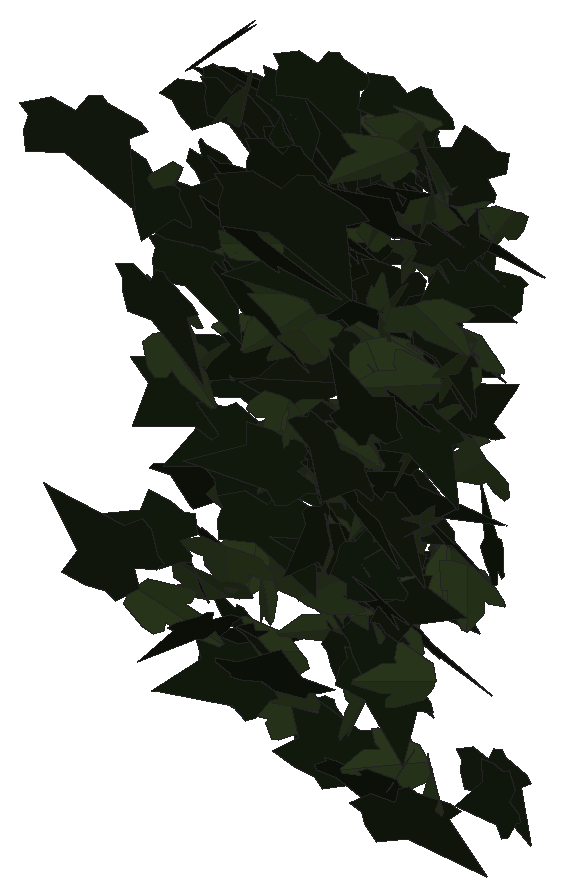
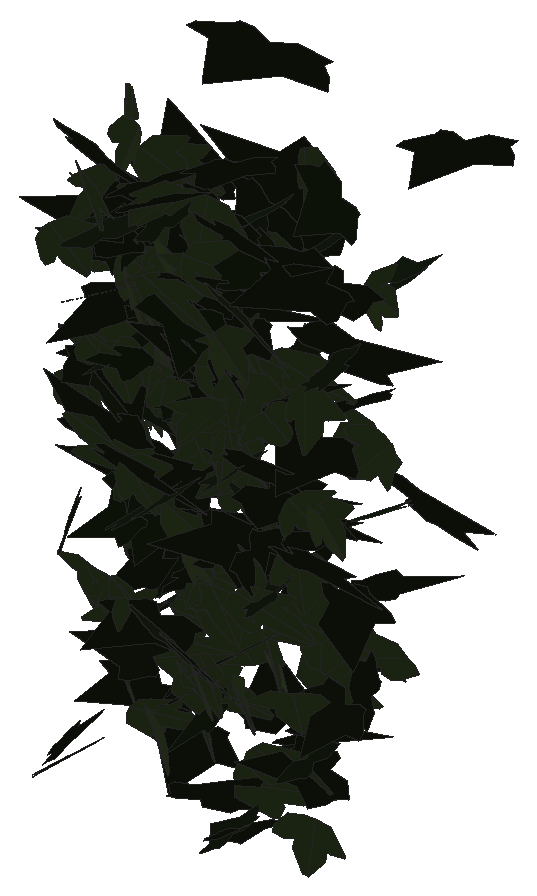
# SketchUp Ruby script. Lengths in millimetres.
U = 1.mm
M = Sketchup.active_model
def pt(a) = Geom::Point3d.new(a.map { |v| v * U })
def face(e, loops, mat)
  f = e.add_face(loops[0].map { |a| pt(a) })
  loops[1..].each { |l| e.add_face(l.map { |a| pt(a) }).erase! }
  f.material = f.back_material = mat if mat
  f
end
# faces: each face lists its corners as indices into pts; further lists are holes
def faces(e, pts, list, mat = nil) = list.each { |f| face(e, (f[0].is_a?(Array) ? f : [f]).map { |l| l.map { |i| pts[i] } }, mat) }
# xy, xz, yz: faces in a plane at the given z, y or x. An outline is a flat list of corners, or four numbers for a rectangle; further outlines are holes
def ring(l) = l.size == 4 ? [[l[0], l[1]], [l[2], l[1]], [l[2], l[3]], [l[0], l[3]]] : l.each_slice(2).to_a
def flat(e, list, mat, &to3) = list.each { |f| face(e, (f[0].is_a?(Array) ? f : [f]).map { |l| ring(l).map { |u, v| to3.(u, v) } }, mat) }
def xy(e, z, list, mat = nil) = flat(e, list, mat) { |x, y| [x, y, z] }
def xz(e, y, list, mat = nil) = flat(e, list, mat) { |x, z| [x, y, z] }
def yz(e, x, list, mat = nil) = flat(e, list, mat) { |y, z| [x, y, z] }
def lines(e, pts, list) = list.each { |a, b| e.add_line(pt(pts[a]), pt(pts[b])) }
# prism: a flat outline (further loops are holes) pulled along v
def prism(e, loops, v, mat = nil)
  f = face(e, loops, mat); d = Geom::Vector3d.new(v.map { |x| x * U })
  f.pushpull(f.normal.samedirection?(d) ? d.length : -d.length)
end
def box(e, o, s, mat = nil) = prism(e, [[o, [o[0] + s[0], o[1], o[2]], [o[0] + s[0], o[1] + s[1], o[2]], [o[0], o[1] + s[1], o[2]]]], [0, 0, s[2]], mat)
def at(x, y, z, deg = 0) = Geom::Transformation.translation(pt([x, y, z])) * Geom::Transformation.rotation(ORIGIN, Z_AXIS, deg.degrees)
def axes(o, x, y, z) = Geom::Transformation.new([*x, 0, *y, 0, *z, 0, *pt(o).to_a, 1])
def part(name) = M.definitions.add(name)
# library, detail: a bought-in or finely detailed component or shape, given as its bounding box
def library(name, o, s) = part(name).tap { |d| box(d.entities, o, s) }
def detail(e, o, s) = box(e.add_group.entities, o, s)
def put(e, d, t, mat = nil) = e.add_instance(d, t).tap { |i| i.material = mat if mat }
def group(e, t, mat = nil) = e.add_group.tap { |g| g.transformation = t; g.material = mat if mat }.entities
root = M.entities
M.materials.add("efeu1").color = [18, 25, 13]
M.materials.add("efeu2").color = [43, 57, 29]
c1 = part("ivyleaf_10")
p = [[0,12.8,-0.8],[-1.5,51.3,-10.9],[-4.9,51,-11.6],[-13.6,26.5,-7.3],[-13.2,15.9,-4.6],[-21.1,19.3,-7.2],
  [-29.5,16.3,-8.3],[-29.2,8.3,-6.2],[-19.7,-9.8,0.5],[-7.6,-13,4],[1,-12.2,5.8],[-0.4,51.1,-11.1],
  [-1.5,51.1,-10.9],[1,-12.4,5.9],[16.9,-12.4,3.5],[35.1,9.1,-5.1],[35,12.9,-6.1],[20.5,16.4,-4.9],
  [15.8,15,-3.8],[15.3,27.6,-7.1],[12.8,31.3,-7.8]]
faces(c1.entities,p,[[0,1,2,3,4,5,6,7,8,9,10],[11,12,0,13,14,15,16,17,18,19,20]],"efeu2")
c2 = part("ivyleaf_9")
p = [[39.1,54.8,31.7],[34.5,51.8,30.2],[-5.3,25.2,17.3],[-17.9,28.3,20.9],[-21.6,21.7,17],[-20.2,4.3,5.3],
  [-22.9,-0.3,2.5],[-17.1,-4,-0.6],[-2,-2.1,-1.2],[-0.7,-15.4,-10.1],[16.6,-22.3,-16.7],[21.1,-15.1,-12.5],
  [32.7,-10.7,-11],[46.1,-1.8,-6.6],[30.8,11.2,3.8]]
faces(c2.entities,p,[[0,1,2,3,4,5,6,7,8,9,10,11,12,13,14]],"efeu1")
put(root,c1,axes([4543,678,3138.6],[-1.58193,0.83154,-0.42194],[0.58084,-0.2915,-1.17569],[-1.67692,-0.88541,-0.00919]))
put(root,c2,axes([4588.4,773.9,3017.7],[-2.04189,0.02362,0.17491],[-0.33312,-0.00391,-1.0731],[-0.04317,-1.08703,0.00766]))
put(root,c2,axes([4606.5,683.4,3248.6],[-0.26226,0.22071,1.22906],[-2.23046,0.404,-0.20395],[-0.8204,-1.16891,0.16157]))
put(root,c2,axes([4552.5,734,2811.4],[1.82354,-0.20517,-0.47825],[-0.87023,0.14656,-0.97893],[0.47292,1.06079,0.04275]))
put(root,c2,axes([4543.6,748.2,3283.7],[1.23051,-0.828,-0.4397],[-0.38091,0.39991,-1.04736],[1.74312,0.67189,0.08152]))
put(root,c1,axes([4575.2,767.9,2648.4],[-1.90726,0.31844,0.17004],[-0.30872,0.051,-1.05151],[-0.61377,-1.01518,0.00051]))
put(root,c2,axes([4537.2,702.8,2816.5],[0.74967,-0.34619,-1.19939],[2.1006,-0.49105,0.50421],[-1.11007,-1.163,0.14414]))
put(root,c2,axes([4581.6,675.2,3027.2],[-1.24627,-0.64137,0.7681],[-0.4534,-0.79163,-0.86412],[1.8497,-0.62618,0.3057]))
put(root,c1,axes([4579.2,767.7,3230.3],[-0.5778,-1.08084,-0.38707],[0.14495,0.38054,-1.12231],[2.18017,-0.31175,-0.02797]))
put(root,c1,axes([4585.8,734,3058.8],[-0.07425,-1.08579,0.28514],[-0.03125,-0.28473,-1.08647],[2.13631,-0.0419,-0.00598]))
put(root,c2,axes([4552.8,739.9,3387.1],[0.13799,-0.32705,-1.15112],[0.68535,1.10574,-0.29147],[2.17196,-0.32813,0.16511]))
put(root,c1,axes([4580.9,639.1,3320.3],[0.20368,-0.86346,0.89476],[0.52681,-0.85899,-0.86205],[2.30715,0.27237,0.11785]))
put(root,c2,axes([4566.5,488.5,3464.7],[-0.43438,-1.01787,-0.89838],[0.34428,0.88006,-1.04307],[2.5608,-0.29098,-0.01215]))
put(root,c2,axes([4575.9,613.6,3327.7],[-0.59648,-0.98235,0.68898],[0.03231,-0.71566,-1.01265],[2.28337,-0.24649,0.19431]))
put(root,c2,axes([4599.1,686,2926.4],[1.22379,0.74994,-0.59671],[-0.79032,-0.42959,-0.98739],[-1.64384,0.76484,0.03049]))
put(root,c2,axes([4618.7,599.2,2886.3],[-0.86103,-0.01575,1.0083],[-1.64942,-0.55895,-0.39759],[0.98126,-0.95338,0.21644]))
put(root,c2,axes([4570.8,692.8,3200.3],[0.10671,-1.19416,-0.39132],[0.1469,0.39424,-1.19202],[2.38712,0.02912,0.09085]))
put(root,c2,axes([4586.6,736.4,3163.5],[1.65295,0.72592,0.00561],[0.0086,0.00335,-1.13194],[-1.3816,0.86852,-0.00033]))
put(root,c2,axes([4564.4,759.5,3393.3],[2.16142,0.05518,0.26359],[0.50154,0.00784,-1.13701],[-0.10567,1.16584,-0.00483]))
put(root,c2,axes([4595.4,689.4,3465.5],[0.63579,0.74247,0.95484],[0.67931,0.88596,-0.81379],[-2.19947,0.48825,0.02467]))
put(root,c1,axes([4599.4,762.2,3076.5],[-0.59048,-0.8322,0.71685],[0.42812,-0.77725,-0.80496],[2.04612,-0.07753,0.3753]))
put(root,c1,axes([4621.6,673.6,2786.3],[-1.68313,-0.18792,-0.61587],[-0.96086,-0.44705,0.86138],[-0.76061,0.98059,0.27467]))
put(root,c1,axes([4623.6,727.9,2973.4],[-1.052,-0.93491,-0.06473],[0.04904,0.05996,-1.08606],[1.7829,-0.55329,-0.00832]))
put(root,c2,axes([4613.3,748.2,3215.6],[-0.75152,-1.04404,0.26644],[-0.20737,-0.24363,-1.11612],[2.0402,-0.40934,-0.0153]))
put(root,c1,axes([4613.3,749.5,2803.8],[1.57621,0.62267,-0.15147],[-0.20029,-0.11201,-1.03583],[-1.20306,0.83445,-0.02601]))
put(root,c2,axes([4665.5,458.4,2930.9],[-2.06405,0.06241,-0.80267],[-1.52815,0.01453,1.08601],[0.11193,1.34916,0.02543]))
put(root,c2,axes([4598.8,707.9,2695.6],[0.35202,0.71468,-0.82032],[0.0774,0.82697,0.72964],[2.06919,-0.15252,0.11226]))
put(root,c1,axes([4613.4,726.1,3186.5],[-0.63082,1.06439,-0.19666],[0.13514,-0.18385,-1.11473],[-2.0556,-0.33872,-0.01293]))
put(root,c1,axes([4657.8,718.8,3229],[0.93414,0.12753,-1.01683],[-1.92982,-0.10292,-0.50236],[-0.2826,1.1244,0.06935]))
put(root,c1,axes([4598.7,741.9,3218.9],[-0.82622,0.33455,-1.04055],[1.21718,-0.83021,-0.53374],[-1.68695,-0.76287,0.12453]))
put(root,c1,axes([4588.3,626.6,3111.4],[1.34835,-0.17595,0.94708],[1.77036,-0.1805,-0.72937],[0.47634,1.16889,0.02993]))
put(root,c2,axes([4648,747.1,3075.7],[-0.01518,0.23814,-1.12079],[-0.44844,-1.0972,-0.23145],[-2.1341,0.22887,0.05661]))
put(root,c1,axes([4633.6,776.7,3192.4],[0.54211,0.89749,-0.56787],[-0.73234,-0.46079,-0.92125],[-1.88397,0.43737,0.19471]))
put(root,c2,axes([4597,739,2721.3],[0.71859,-0.97928,0.3703],[0.41503,-0.31145,-1.046],[1.94886,0.42741,0.08622]))
put(root,c1,axes([4591.2,592.3,2800.7],[0.8964,0.2162,0.97025],[1.6901,0.39094,-0.5182],[-0.85013,1.00518,-0.00715]))
put(root,c2,axes([4606.6,718.4,3400.2],[0.47706,-1.1436,0.04901],[0.00765,-0.04929,-1.17073],[2.17849,0.2506,-0.00662]))
put(root,c1,axes([4666.3,733.7,2698.9],[-0.98064,0.01279,0.89908],[-1.47187,-0.53494,-0.4356],[0.87303,-0.88751,0.27551]))
put(root,c1,axes([4645.7,661,2848.3],[-2.04059,-0.16162,0.08184],[-0.15185,-0.01977,-1.08427],[0.30954,-1.07513,0.00763]))
put(root,c2,axes([4661.4,677.6,2998.2],[-1.70018,-0.43925,0.45376],[-0.66037,-0.31541,-0.98843],[1.00428,-0.95103,0.11824]))
put(root,c1,axes([4672.6,759,2918.6],[-1.02752,-0.21117,0.91697],[-1.42909,-0.54043,-0.56656],[1.07927,-0.91665,0.12279]))
put(root,c1,axes([4620,711.2,2884.1],[-0.68337,-0.57703,0.9887],[1.15406,0.78302,0.67721],[-1.84796,0.70238,0.0573]))
put(root,c2,axes([4673.6,664.4,2697.8],[-1.32992,-0.4501,0.85865],[-1.25427,-0.55574,-0.82765],[1.35322,-0.95746,0.07674]))
put(root,c2,axes([4687.5,774.7,3119.1],[-2.04699,-0.09835,0.22206],[-0.41345,-0.06118,-1.07929],[0.20666,-1.09653,0.0403]))
put(root,c1,axes([4699.2,715.9,2644.9],[-0.06533,0.03688,-1.24408],[-2.21027,-0.44855,0.01875],[-0.85192,1.16091,0.04677]))
put(root,c2,axes([4680.6,582.9,2808.3],[-0.57562,0.60142,-0.88442],[0.19749,-0.89826,-0.64632],[-2.02593,-0.25844,0.18828]))
put(root,c2,axes([4634.2,737.6,3362.5],[0.96968,-1.08808,0.14521],[0.11602,-0.1318,-1.20146],[2.08597,0.51313,-0.00068]))
put(root,c2,axes([4649.5,680.5,2954.9],[0.60981,-0.95034,-0.85727],[-0.55424,0.80641,-1.00281],[2.37195,0.43275,-0.01392]))
put(root,c2,axes([4641.8,754.4,2944.4],[1.04178,-0.96438,-0.08653],[-0.04623,0.08569,-1.1087],[1.8422,0.54752,0.02111]))
put(root,c2,axes([4642.7,527.9,3253.3],[0.68393,-1.31283,-0.03189],[-0.01948,0.03026,-1.36113],[2.49924,0.3595,-0.00188]))
put(root,c1,axes([4672.4,767.1,3220.9],[-1.07092,-0.94805,-0.32511],[0.41799,0.24715,-1.10082],[1.86112,-0.60103,0.06016]))
put(root,c2,axes([4680.7,743.6,2979.8],[-0.47406,0.25077,-1.09909],[0.74862,-1.03553,-0.32541],[-2.01071,-0.44467,0.13797]))
put(root,c1,axes([4678.5,713.4,2845.2],[0.89008,-0.92506,-0.4502],[-0.1471,0.46154,-1.02866],[1.95246,0.45648,0.12773]))
put(root,c1,axes([4670.1,781.1,2803.5],[0.94415,-0.91619,0.26202],[0.28525,-0.2167,-1.04151],[1.79103,0.51749,0.02775]))
put(root,c1,axes([4678.1,643.1,3464.8],[0.02137,-1.16228,-0.38586],[0.1283,0.38588,-1.16037],[2.32722,-0.0106,0.06751]))
put(root,c1,axes([4661.2,713.2,2788.2],[-0.56556,0.049,-1.06746],[0.45682,-1.07659,-0.11624],[-1.98176,-0.26215,0.27784]))
put(root,c1,axes([4700.3,697.4,3195.4],[-1.21986,-0.81554,0.40318],[-0.50925,-0.30239,-1.03704],[1.65487,-0.69421,-0.02193]))
put(root,c2,axes([4674.6,772.7,2617.8],[-0.51151,-0.98309,0.00849],[0.00873,-0.01006,-1.01914],[1.87107,-0.26871,0.00708]))
put(root,c1,axes([4695.2,783.7,3272.6],[-0.06078,-1.05145,0.41917],[0.0409,-0.41982,-1.05145],[2.15388,-0.0217,0.03179]))
put(root,c2,axes([4724.8,752.1,3317.8],[-1.07947,0.89986,0.44017],[-0.51038,0.35098,-1.06306],[-1.83694,-0.62631,0.0367]))
put(root,c2,axes([4660.8,650.3,3213.9],[1.55261,-1.023,-0.08756],[-0.09223,0.07335,-1.30842],[1.95191,0.81719,0.00782]))
put(root,c1,axes([4698.4,727.9,2958],[0.01329,-0.3992,1.07691],[0.09042,-1.07591,-0.39914],[2.18399,0.04697,0.00997]))
put(root,c1,axes([4691.6,703.7,3187.5],[0.23506,-0.31709,-1.15718],[0.66422,1.12249,-0.27033],[2.1848,-0.30714,0.20669]))
put(root,c2,axes([4722,757.2,3411.1],[-2.19236,0.12858,-0.12998],[0.24963,0.00352,-1.15895],[-0.24241,-1.15924,-0.01793]))
put(root,c1,axes([4692.5,746.6,3255.4],[0.12653,-0.35323,1.09107],[0.662,-1.03521,-0.35634],[2.07983,0.35099,0.04704]))
put(root,c2,axes([4685.9,732,3425.7],[-0.02998,-1.11088,0.30737],[-0.02421,-0.30721,-1.11097],[2.19354,-0.01857,-0.00806]))
put(root,c2,axes([4681.3,772.7,3104.5],[0.5072,-1.08797,-0.04092],[-0.01495,0.04021,-1.12013],[2.07204,0.26661,0.00194]))
put(root,c1,axes([4715.9,751.9,3139.5],[-1.5463,-0.56729,0.53644],[-0.23826,-0.66952,-0.89765],[1.46672,-0.70684,0.41973]))
put(root,c2,axes([4663.7,758.5,3374.7],[0.87099,-0.77691,0.66757],[1.02335,-0.44012,-0.88083],[1.65931,0.67925,0.19282]))
put(root,c1,axes([4705.6,762.6,3124.4],[-0.21582,-1.00262,-0.50322],[0.21706,0.49286,-1.00767],[2.12397,-0.15224,0.05185]))
put(root,c2,axes([4684.3,780,2611],[0.22121,-1.01794,0.40978],[0.06159,-0.40871,-1.02447],[2.08752,0.11993,-0.0132]))
put(root,c1,axes([4726.8,684.4,3177],[-1.09429,-0.71135,0.88246],[-0.56582,-0.86022,-0.88713],[2.08169,-0.60775,0.22276]))
put(root,c1,axes([4722.8,758.1,3254.7],[1.17445,0.63757,-0.66256],[-1.15457,-0.31734,-0.87038],[-1.3151,0.84799,0.17244]))
put(root,c1,axes([4688.9,746.7,2958],[-1.31286,0.44031,-0.73253],[1.00453,-0.52093,-0.81016],[-1.27937,-0.86085,0.11558]))
put(root,c2,axes([4743.8,653.8,2995.5],[-1.40461,-0.1095,0.82678],[-1.402,-0.43203,-0.71479],[0.7442,-1.02059,0.21388]))
put(root,c2,axes([4692.4,766,2844.8],[-0.02671,-1.35925,0.1072],[-0.01214,-0.10714,-1.35931],[2.59493,-0.01449,-0.00526]))
put(root,c1,axes([4742.5,688.4,3019.4],[-1.45531,0.17773,0.774],[-1.45613,0.12307,-0.78413],[-0.40503,-1.08104,0.03798]))
put(root,c1,axes([4708.6,677.8,3049.2],[1.70359,-0.62561,0.1387],[0.21653,-0.07933,-1.09207],[1.2002,0.90232,0.00015]))
put(root,c2,axes([4700.6,657.5,2706.9],[1.97972,0.12419,0.34433],[-0.64967,-0.04538,1.04759],[0.2515,-1.09478,-0.00437]))
put(root,c1,axes([4741.1,762.5,3358.5],[-0.38221,-0.48441,1.10209],[-0.97687,-0.97622,-0.52262],[2.07249,-0.54948,-0.04309]))
put(root,c1,axes([4735.3,751.2,2901],[-1.81645,0.28591,0.35961],[-0.80795,-0.23189,-0.94233],[-0.33426,-0.99321,0.32353]))
put(root,c2,axes([4753.7,698.6,3072.2],[-1.4024,0.65635,0.50313],[-0.68168,0.35411,-0.98652],[-1.41867,-0.81897,-0.02333]))
put(root,c2,axes([4692.1,733.9,2979.5],[0.29604,0.57908,-0.98023],[0.46911,0.94874,0.59959],[2.1154,-0.29143,0.00421]))
put(root,c1,axes([4716.3,791.2,3238.5],[0.00274,-0.4635,1.03889],[0.65548,-0.98996,-0.44215],[2.06346,0.31509,0.13907]))
put(root,c2,axes([4712.7,727.8,3277],[2.13743,0.05674,-0.42471],[-0.81221,0.04132,-1.12297],[-0.0731,1.19998,0.05875]))
put(root,c1,axes([4731,753.1,3152.9],[-1.73179,-0.65821,-0.11627],[0.17511,0.07119,-1.12304],[1.25999,-0.91457,-0.00374]))
put(root,c1,axes([4753.9,752.9,2801.5],[-1.22778,0.36869,0.73526],[-1.26518,0.31657,-0.74201],[-0.92187,-0.9255,0.03909]))
put(root,c1,axes([4751.8,742.5,3136.5],[-1.96727,-0.04626,0.44618],[-0.82971,-0.16035,-1.0266],[0.20106,-1.11438,0.12919]))
put(root,c2,axes([4710.3,724.8,3371],[0.33563,-0.89983,0.73727],[0.38895,-0.71014,-0.91559],[2.17955,0.26529,0.04986]))
put(root,c1,axes([4770.8,735.8,2766.9],[-0.69405,-0.36654,1.07429],[-1.43227,-0.76666,-0.51704],[1.61728,-0.83626,0.00314]))
put(root,c1,axes([4723,761.9,3166.5],[0.88975,0.97275,0.52919],[0.4491,0.47371,-1.07924],[-2.05915,0.52364,-0.00672]))
put(root,c2,axes([4723.1,637.9,2945.2],[-0.45857,-0.98827,-0.75141],[0.32867,0.73131,-1.01721],[2.33983,-0.29641,-0.00438]))
put(root,c1,axes([4740.2,767.3,2769.9],[1.42289,-0.76272,0.2847],[-0.30747,0.23986,1.06682],[-1.51862,-0.7632,0.05076]))
put(root,c2,axes([4728.9,750.8,2756.6],[1.38102,-0.62599,-0.58774],[-0.77183,0.42843,-0.95699],[1.44046,0.82972,0.05071]))
put(root,c2,axes([4751.9,769.3,3332.3],[-1.77337,-0.60027,-0.16865],[0.23467,0.11987,-1.10789],[1.16324,-0.93931,-0.03361]))
put(root,c2,axes([4778.3,681,3245.5],[-1.39181,-0.24912,0.86653],[-1.45289,-0.42258,-0.76575],[0.91304,-1.05218,0.10239]))
put(root,c2,axes([4728.4,721.8,3480.4],[-0.21372,-1.01707,-0.53891],[0.22963,0.52808,-1.02178],[2.17855,-0.15544,0.05483]))
put(root,c1,axes([4730.8,701.7,2808.3],[-1.48122,-0.54053,0.59136],[0.90767,0.3499,0.94748],[-1.22521,0.91269,-0.01301]))
put(root,c2,axes([4776.5,718.4,2598.9],[-1.99052,-0.62987,0.12428],[0.21361,0.05451,1.22085],[-1.20306,1.05183,0.01115]))
put(root,c2,axes([4775.7,682.8,3037.4],[-1.35997,0.84188,-0.07063],[0.08502,-0.05472,-1.10425],[-1.60564,-0.71596,0.00135]))
put(root,c2,axes([4784.4,763,2819.4],[-1.44688,0.62857,0.34419],[-0.48707,0.23056,-0.98634],[-1.27396,-0.80204,-0.0138]))
put(root,c1,axes([4734.8,685.7,3045.1],[0.63235,0.53253,0.91579],[0.49157,0.89009,-0.6113],[-1.95534,0.39599,0.14248]))
put(root,c1,axes([4745.8,715,2912],[0.35061,0.48753,0.98825],[-0.05603,1.00379,-0.48971],[-2.09652,0.0547,0.17836]))
put(root,c2,axes([4702,601.4,3314.5],[1.27843,-0.69409,0.94764],[1.33702,-0.63752,-0.96491],[1.7917,0.97099,0.04387]))
put(root,c2,axes([4735.8,779.1,3239.7],[-1.21742,-0.32249,-0.87641],[1.65424,0.18286,-0.70168],[0.64993,-1.0695,0.1443]))
put(root,c1,axes([4762.3,737.8,3416.1],[-2.1634,0.1388,0.06251],[-0.11987,-0.00011,-1.14513],[-0.26376,-1.13843,0.00773]))
put(root,c2,axes([4736,728.5,3416],[-1.14395,-0.14295,-0.98246],[1.86084,0.11407,-0.61478],[0.3279,-1.14608,0.06136]))
put(root,c2,axes([4732.9,651.4,3394.7],[-1.08916,-0.08517,-1.08809],[2.06228,0.1026,-0.57794],[0.24843,-1.22512,0.02724]))
put(root,c2,axes([4762.2,753.9,3281.1],[0.95514,0.98803,0.08297],[-0.0259,0.09985,-1.10671],[-1.88687,0.49877,0.05719]))
put(root,c1,axes([4761.6,761.3,2962.1],[0.2858,-0.99933,0.54967],[0.2761,-0.53318,-1.00898],[2.15302,0.20103,0.05642]))
put(root,c2,axes([4777.2,758.5,2917.4],[-0.09868,-0.87247,-0.6914],[0.18524,-0.69305,0.86725],[-2.11055,-0.02003,0.10844]))
put(root,c1,axes([4757.5,658.1,3172.4],[-0.9297,-0.88996,-0.6184],[0.76074,0.48254,-1.01018],[1.91713,-0.62306,0.10096]))
put(root,c1,axes([4744.2,632.2,3330.6],[-1.89349,-0.17353,-0.76084],[1.41716,0.15784,-1.00968],[0.44448,-1.24249,-0.022]))
put(root,c2,axes([4737.2,740.7,3219.1],[0.11589,-0.01892,1.14687],[2.05985,0.38125,-0.05117],[-0.72288,1.08335,0.03804]))
put(root,c2,axes([4799.7,687.2,3149.8],[-2.07169,-0.02079,0.21967],[-0.41686,-0.03195,-1.08839],[0.05081,-1.11002,0.02721]))
put(root,c1,axes([4803.2,770.9,3309.3],[1.35035,-0.23046,-0.83576],[-1.47887,0.30988,-0.74512],[0.73171,1.05161,0.03641]))
put(root,c2,axes([4779.8,692.6,3205.2],[1.85272,0.50571,-0.51933],[-0.88589,-0.23049,-1.09695],[-1.05757,1.079,0.00908]))
put(root,c2,axes([4738,586.5,3377.8],[0.75403,-0.63871,1.19356],[1.61484,-0.85186,-0.7375],[2.0075,0.92514,0.14494]))
put(root,c2,axes([4786.3,790.2,3027.8],[-0.33821,-0.91212,0.58358],[-0.16364,-0.57763,-0.92901],[2.05434,-0.19618,0.02207]))
put(root,c2,axes([4773.2,705.2,2912.6],[0.20911,-0.70699,0.90466],[0.36283,-0.88494,-0.71474],[2.15482,0.21762,0.03256]))
put(root,c2,axes([4829.6,760.4,2843.9],[-1.24567,0.806,0.14383],[-0.28188,0.06454,-1.03567],[-1.5325,-0.66702,0.07359]))
put(root,c1,axes([4831.5,717.7,2769.4],[1.43347,0.28695,0.9196],[-1.65345,-0.30202,0.8058],[0.79215,-1.14967,0.01784]))
put(root,c1,axes([4807.2,692.5,2701.9],[0.88514,-1.09845,-0.15462],[-0.07744,0.15065,-1.19266],[2.10975,0.46638,0.02109]))
put(root,c2,axes([4793.1,687.7,2781.1],[0.6588,-0.72376,-0.75846],[-0.63985,0.67991,-0.80224],[1.88988,0.48249,-0.00722]))
put(root,c1,axes([4793.7,688.7,3064.9],[-1.71273,0.46871,-0.43556],[0.69478,-0.24119,-1.01382],[-1.00011,-0.97026,0.04161]))
put(root,c2,axes([4792,738.8,2741.9],[-0.11149,-1.09476,0.14406],[-0.02759,-0.14349,-1.09631],[2.10133,-0.05997,-0.00675]))
put(root,c1,axes([4842.4,693.7,3211.8],[-0.04692,0.1348,1.21745],[-1.90127,0.70242,-0.09801],[-1.34898,-0.99469,0.09578]))
put(root,c2,axes([4818.3,768.4,3417.9],[-1.07236,-0.92631,0.35645],[-0.22944,-0.34298,-1.08186],[1.87499,-0.57175,0.07148]))
put(root,c1,axes([4822,751.6,3192.9],[-0.27773,0.73905,-0.88205],[-0.29294,-0.89366,-0.72332],[-2.17042,0.02605,0.21049]))
put(root,c2,axes([4805.3,756.7,3385.6],[-0.02373,-0.83516,0.7987],[0.12508,-0.79797,-0.83336],[2.19578,0.03643,0.0561]))
put(root,c1,axes([4806.8,742.6,3421.9],[1.00469,0.94038,0.57255],[0.55162,0.49386,-1.07837],[-2.02144,0.60215,-0.00971]))
put(root,c1,axes([4830.9,707.1,2966.6],[-0.05124,-0.8716,0.71638],[0.08983,-0.71683,-0.87037],[2.14535,0.0092,0.05355]))
put(root,c1,axes([4814.5,648.7,3059],[-0.65707,-0.70898,-0.784],[0.99921,0.60081,-0.77452],[1.74604,-0.61063,0.14821]))
put(root,c2,axes([4814.4,772.8,3449.7],[-0.32844,-1.1516,-0.10953],[-0.01396,0.11183,-1.16422],[2.20157,-0.17109,-0.02372]))
put(root,c1,axes([4829.6,728.3,3340],[0.49209,-0.98732,0.57844],[0.21855,-0.56764,-1.02021],[2.16681,0.28148,-0.02846]))
put(root,c2,axes([4799.7,684.7,2990.1],[-0.31952,-0.03446,1.18247],[2.22703,0.1705,0.17111],[-0.33054,1.18209,0.00979]))
put(root,c2,axes([4868,725.6,3233.5],[-0.05671,-0.03397,-1.17134],[-1.58218,-0.82519,0.04508],[-1.57181,0.83186,-0.00312]))
put(root,c1,axes([4809.6,726.2,3310.5],[-0.27994,-0.36555,-1.08993],[1.38165,0.82246,-0.37382],[1.69647,-0.73016,0.1246]))
put(root,c1,axes([4838.1,730.1,3226.2],[0.49353,-1.16142,0.20107],[0.06513,-0.19838,-1.18998],[2.24236,0.26139,-0.00969]))
put(root,c1,axes([4857.5,689.6,3425.2],[-0.75815,-0.58287,0.93557],[-0.77296,-0.8472,-0.70074],[1.95029,-0.56236,0.08597]))
put(root,c2,axes([4872.7,773.3,3054.3],[-1.90553,0.27768,0.37939],[-0.70515,0.08348,-1.03887],[-0.55085,-1.06744,0.01745]))
put(root,c1,axes([4848,761.7,3039],[-0.44215,-1.01093,0.29277],[-0.14985,-0.28228,-1.0372],[1.99745,-0.24495,-0.01301]))
put(root,c2,axes([4817.8,755.1,2848.3],[-0.30335,-0.3452,-1.08523],[0.70209,1.02107,-0.37897],[2.05051,-0.40068,-0.03079]))
put(root,c1,axes([4830.4,723.7,3148.6],[2.01287,0.28651,0.17736],[0.31486,0.06746,-1.09553],[-0.55869,1.07027,0.02158]))
put(root,c1,axes([4854.2,719.2,3446.2],[-0.37318,-0.82391,0.82247],[-0.02902,-0.83217,-0.83726],[2.21545,-0.14969,0.12757]))
put(root,c2,axes([4887.8,653.2,2910.2],[-0.70635,-0.06817,1.16218],[-2.18582,-0.1781,-0.37722],[0.36244,-1.20693,-0.00998]))
put(root,c2,axes([4843,650.3,2638.8],[1.83505,0.41931,-0.38004],[-0.67401,-0.13853,-1.05134],[-0.84008,1.02709,0.01335]))
put(root,c1,axes([4816.7,706.6,3172.2],[-1.14848,-0.21094,-0.91125],[1.77972,-0.11218,-0.59329],[0.03919,-1.08717,0.23802]))
put(root,c1,axes([4828.4,672.3,2807.5],[-0.72051,0.38595,-0.95882],[0.85086,-0.8595,-0.5225],[-1.77358,-0.56913,0.13886]))
put(root,c2,axes([4844,589.7,2985.5],[0.01612,-0.3251,-1.17649],[1.25671,-0.98827,0.27784],[-1.95372,-0.63837,0.16901]))
put(root,c2,axes([4818.7,702.5,3141.8],[1.73859,-0.89137,-0.01362],[-0.01578,0.011,-1.27633],[1.69657,0.91354,0.00208]))
put(root,c1,axes([4857.5,752.9,3290.3],[0.3014,-1.1301,-0.14598],[-0.0106,0.14661,-1.14105],[2.16865,0.15778,0.01471]))
put(root,c2,axes([4841.6,643.1,2889.7],[1.92503,-0.09508,-0.43493],[-0.81216,0.10069,-1.01442],[0.24152,1.09641,0.05545]))
put(root,c1,axes([4845.1,673.7,3170.3],[0.71786,1.09901,0.16166],[0.07492,0.15739,-1.16186],[-2.11282,0.37899,0.01372]))
put(root,c1,axes([4870.1,560.8,2979.3],[0.16084,-0.44052,-1.03923],[-0.28999,1.02815,-0.44822],[2.12856,0.17336,0.01746]))
put(root,c2,axes([4826.8,694.8,3358.9],[1.95636,0.37138,0.65667],[1.12158,0.29764,-1.09083],[-0.89643,1.18291,0.06831]))
put(root,c1,axes([4850.7,734.2,3206.9],[-1.64048,-0.52468,-0.46844],[0.99834,0.01409,-0.98099],[0.89181,-0.98093,0.23648]))
put(root,c1,axes([4870.9,741.3,3298.9],[-0.1392,-1.11185,0.34435],[-0.026,-0.34419,-1.11422],[2.21508,-0.07391,0.00856]))
put(root,c1,axes([4888.1,720.2,3278.9],[-1.71134,0.64453,-0.4114],[-0.67357,0.21212,1.10588],[1.28998,0.96582,0.03166]))
put(root,c1,axes([4891.9,680.2,2657.9],[-0.73481,0.02502,0.98744],[-0.96697,-0.91421,-0.1755],[1.61213,-0.53695,0.34481]))
put(root,c1,axes([4888.6,749.9,3187],[-2.0576,0.1071,0.42641],[-0.8127,0.01361,-1.08609],[-0.19915,-1.1621,0.02658]))
put(root,c2,axes([4882.7,741.7,2950.2],[0.12129,-1.18239,-0.08417],[0.06785,-0.08234,1.1837],[-2.25499,-0.06607,0.03109]))
put(root,c2,axes([4861,591.5,3088.9],[-0.63959,-0.8834,0.86363],[-0.03142,-0.89172,-0.91856],[2.35102,-0.25224,0.22267]))
put(root,c2,axes([4837.4,626.6,3025.4],[0.62295,-1.16137,0.69855],[0.57614,-0.63782,-1.20226],[2.51417,0.43392,0.10242]))
put(root,c1,axes([4880.5,685.2,2657.7],[0.58573,-1.12767,-0.29822],[-0.15866,0.28638,-1.1689],[2.21429,0.31882,-0.00487]))
put(root,c2,axes([4847.6,637.5,3373.7],[2.33819,-0.19127,-0.04988],[0.09596,-0.00036,1.24333],[-0.36376,-1.22957,0.00739]))
put(root,c2,axes([4837.8,745.2,2784.2],[1.22444,-0.67956,0.58735],[0.81048,-0.40534,-0.93543],[1.50512,0.77109,0.0259]))
put(root,c2,axes([4886.8,670.2,2949.1],[0.56417,1.14778,0.66283],[0.32388,0.64062,-1.18543],[-2.50166,0.34178,-0.00399]))
put(root,c2,axes([4858.6,652.7,2823.2],[0.87182,-1.01494,-0.46328],[-0.20753,0.45768,-1.11049],[2.11318,0.46368,0.08207]))
put(root,c1,axes([4863.4,778.3,2869.9],[-0.96674,0.43245,-0.82649],[0.90413,-0.68996,-0.65298],[-1.5278,-0.68195,0.13655]))
put(root,c1,axes([4879.3,747.8,2835.2],[0.9178,0.98953,-0.45958],[0.3321,0.42605,1.10044],[2.04976,-0.5121,0.02749]))
put(root,c2,axes([4849.7,750.7,3201.8],[1.76199,-0.63304,0.22891],[0.33288,-0.14967,-1.12128],[1.23715,0.94187,-0.02432]))
put(root,c2,axes([4909.8,585.6,3136.7],[0.3657,0.06858,1.11893],[-0.87963,1.03912,0.01568],[-1.94378,-0.45734,0.20342]))
put(root,c2,axes([4907.6,734.5,3134.9],[-1.18224,0.66692,-0.67679],[0.45085,-0.67436,-0.88194],[-1.75127,-0.62383,0.22984]))
put(root,c2,axes([4880.7,672.4,2866.4],[0.29887,0.04249,-1.1026],[-0.58306,1.0716,-0.00234],[2.01745,0.30341,0.16267]))
put(root,c1,axes([4873.4,751.3,3051.6],[-0.99308,-0.69168,0.777],[0.80832,0.65186,0.86551],[-1.80729,0.67162,-0.03984]))
put(root,c2,axes([4846,685.4,2993.2],[1.04954,0.37113,-0.99817],[1.41015,0.67368,0.65982],[1.45579,-0.92012,0.08049]))
put(root,c2,axes([4875,654,3140.8],[2.03347,-0.15647,-0.28734],[-0.53921,0.04837,-1.07983],[0.31145,1.10536,0.00658]))
put(root,c2,axes([4905.5,735.4,3157.3],[0.56572,0.91516,-0.57383],[-0.26283,-0.55808,-0.96158],[-2.03894,0.32586,-0.03526]))
put(root,c1,axes([4914.9,668.6,3161],[0.03154,-0.06122,1.22241],[-0.72755,-1.16162,-0.05299],[2.21287,-0.38105,-0.03485]))
put(root,c1,axes([4901.6,683,2973.2],[-0.75714,-1.11946,-0.31869],[0.15984,0.30831,-1.18782],[2.20944,-0.40593,-0.02328]))
put(root,c2,axes([4877.3,651.2,2999.3],[0.50846,-1.10871,-0.01815],[-0.00182,0.01844,-1.14043],[2.11037,0.26714,0.00339]))
put(root,c2,axes([4897.4,769.6,3265.9],[-0.9496,-0.93329,0.44428],[-0.0599,-0.47939,-1.04238],[1.96632,-0.46532,0.18281]))
put(root,c2,axes([4875.2,726.7,2954.7],[1.58081,-0.71632,-0.10791],[-0.12474,0.08919,-1.09655],[1.37302,0.83283,0.02462]))
put(root,c2,axes([4889.3,727.4,3241.2],[0.20634,-0.01626,-1.24294],[-0.39483,1.22992,-0.03418],[2.33258,0.20963,0.10417]))
put(root,c2,axes([4879.1,470,3480.7],[-1.13076,-0.71943,-1.18347],[1.5114,0.87809,-0.93247],[2.15955,-0.99125,0.03293]))
put(root,c1,axes([4908.4,671.2,3082],[0.60686,-1.02934,0.29924],[0.12815,-0.29234,-1.07739],[2.03612,0.32519,-0.02138]))
put(root,c1,axes([4910.2,691,3442.6],[-1.31208,0.91652,0.1856],[-0.23056,0.1411,-1.1468],[-1.76473,-0.69987,0.01184]))
put(root,c2,axes([4884.6,775.6,3351.5],[-0.17151,-1.03828,0.50429],[0.54509,-0.51012,-0.9991],[2.1281,0.04699,0.29655]))
put(root,c2,axes([4892.8,634,2790.8],[-0.1599,-1.27799,0.06757],[-0.00687,-0.06748,-1.28075],[2.43566,-0.08409,0.00083]))
put(root,c2,axes([4883.8,759.4,3073.2],[-0.72647,0.23002,0.98589],[1.62129,-0.49631,0.44562],[1.04103,0.93347,-0.00601]))
put(root,c2,axes([4889.5,743.7,3173.4],[0.20543,-1.10129,0.33816],[0.13936,-0.33239,-1.10589],[2.18813,0.12456,0.03869]))
put(root,c1,axes([4920.7,759.7,3404.5],[1.32132,-0.92357,-0.08588],[0.02142,0.11565,-1.15276],[1.76519,0.68993,0.07827]))
put(root,c2,axes([4889,728.5,3327.6],[1.92919,-0.56525,0.11525],[0.18724,-0.06021,-1.1606],[1.08183,1.01841,-0.00465]))
put(root,c1,axes([4907.4,748.4,3176.5],[2.19185,-0.29752,0.30534],[0.56782,-0.06583,-1.18943],[0.57959,1.18963,0.01055]))
put(root,c2,axes([4967.5,717.7,3423.9],[-1.39519,0.63328,0.67202],[-1.03094,0.39997,-0.96781],[-1.42324,-0.91051,0.04226]))
put(root,c1,axes([4910.9,753.6,2871.1],[1.99179,-0.28369,0.29762],[0.53671,-0.09707,-1.08415],[0.56947,1.08371,-0.0192]))
put(root,c2,axes([4904,724,3194.8],[0.32838,-1.10914,0.18831],[0.11112,-0.18143,-1.1221],[2.13824,0.17976,0.02939]))
put(root,c2,axes([4880.8,730.7,3345.8],[1.59831,-0.54203,0.77215],[1.26422,-0.39434,-0.99927],[1.27497,1.07051,0.02287]))
put(root,c2,axes([4937.4,692.6,3325.2],[-1.53508,0.92435,-0.04216],[-0.08516,0.01691,1.22657],[1.75899,0.8075,0.02259]))
put(root,c1,axes([4920.6,704.8,3380.3],[-1.37208,-0.6999,-0.70225],[1.05352,0.4362,-1.00302],[1.56547,-0.90699,0.05951]))
put(root,c1,axes([4946.8,780.7,3333.9],[-0.72018,-0.93309,0.51895],[-0.15059,-0.52456,-1.00087],[2.02644,-0.3706,0.11005]))
put(root,c1,axes([4947.7,706.5,3188],[0.16312,-1.15597,0.21565],[0.01398,-0.21569,-1.15911],[2.23795,0.0856,-0.00848]))
put(root,c2,axes([4924.5,650.8,3124.1],[0.18823,-1.15522,-0.38831],[-0.06246,0.38692,-1.15945],[2.31866,0.1042,0.00029]))
put(root,c2,axes([4971.3,726.8,3299.8],[-2.03672,-0.40288,0.14132],[-0.25723,-0.04209,-1.14345],[0.77077,-1.07862,-0.00817]))
put(root,c2,axes([4932,774.9,2629],[0.38617,-1.07528,-0.22524],[-0.0564,0.22361,-1.09419],[2.09014,0.2047,0.01209]))
put(root,c1,axes([4965.1,599.2,2825],[-0.07449,0.24254,1.17217],[-0.37437,-1.15816,0.23308],[2.24717,-0.1849,0.07768]))
put(root,c2,axes([4963.9,746.3,2908.5],[-0.17111,-0.69281,0.9551],[0.50794,0.9211,0.69327],[-2.18741,0.26808,0.08627]))
put(root,c1,axes([4940.8,644.8,3271.4],[-1.4293,-0.60655,-0.59353],[1.07242,0.23624,-0.9544],[1.20771,-0.92762,0.14504]))
put(root,c1,axes([4965.3,622.8,3441.8],[0.58839,-0.96914,-0.74002],[0.1185,0.77498,-0.98891],[2.31767,0.20641,0.23843]))
put(root,c1,axes([4991.6,687.8,3075.9],[-1.55469,0.37823,0.76082],[-1.39402,0.22138,-0.89649],[-0.81949,-1.09414,0.08162]))
put(root,c2,axes([4935.4,607.4,2649.5],[-0.22462,-0.3116,-1.076],[1.28323,0.84426,-0.31845],[1.70255,-0.67744,0.09806]))
put(root,c2,axes([4977.5,748.2,2607.3],[-0.45164,-0.26128,1.03907],[-0.93648,-0.91881,-0.34341],[1.81137,-0.54017,0.08153]))
put(root,c1,axes([4947.1,646.7,2668.4],[-0.03945,0.06565,1.12865],[1.49979,-0.80858,0.0615],[1.54282,0.7877,-0.03093]))
